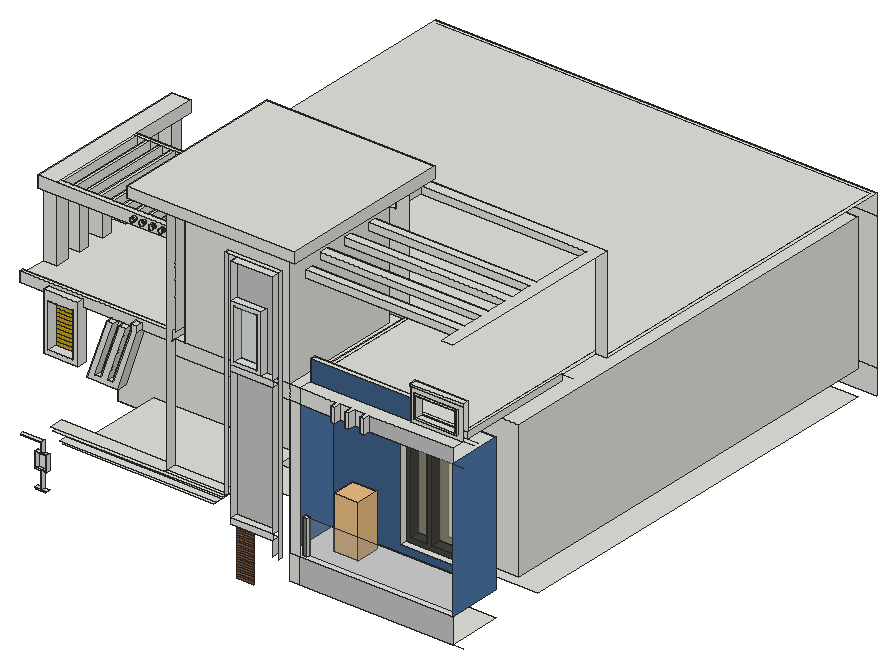
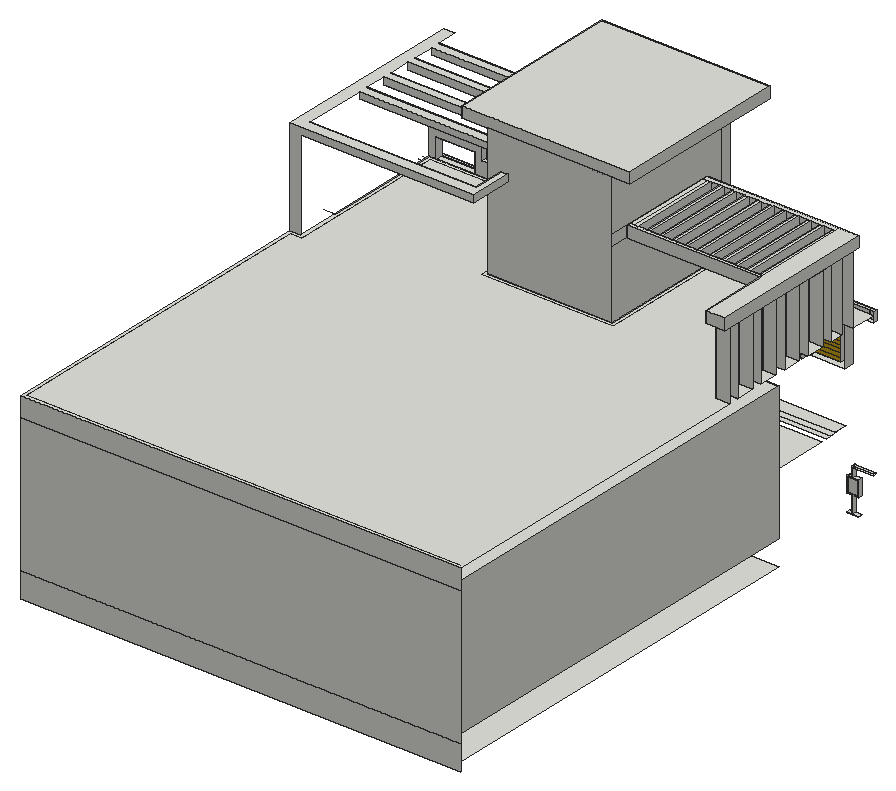
# SketchUp Ruby script. Lengths in inches.
U = 1.inch
M = Sketchup.active_model
def pt(a) = Geom::Point3d.new(a.map { |v| v * U })
def face(e, loops, mat)
  f = e.add_face(loops[0].map { |a| pt(a) })
  loops[1..].each { |l| e.add_face(l.map { |a| pt(a) }).erase! }
  f.material = f.back_material = mat if mat
  f
end
# faces: each face lists its corners as indices into pts; further lists are holes
def faces(e, pts, list, mat = nil) = list.each { |f| face(e, (f[0].is_a?(Array) ? f : [f]).map { |l| l.map { |i| pts[i] } }, mat) }
# xy, xz, yz: faces in a plane at the given z, y or x. An outline is a flat list of corners, or four numbers for a rectangle; further outlines are holes
def ring(l) = l.size == 4 ? [[l[0], l[1]], [l[2], l[1]], [l[2], l[3]], [l[0], l[3]]] : l.each_slice(2).to_a
def flat(e, list, mat, &to3) = list.each { |f| face(e, (f[0].is_a?(Array) ? f : [f]).map { |l| ring(l).map { |u, v| to3.(u, v) } }, mat) }
def xy(e, z, list, mat = nil) = flat(e, list, mat) { |x, y| [x, y, z] }
def xz(e, y, list, mat = nil) = flat(e, list, mat) { |x, z| [x, y, z] }
def yz(e, x, list, mat = nil) = flat(e, list, mat) { |y, z| [x, y, z] }
def lines(e, pts, list) = list.each { |a, b| e.add_line(pt(pts[a]), pt(pts[b])) }
# prism: a flat outline (further loops are holes) pulled along v
def prism(e, loops, v, mat = nil)
  f = face(e, loops, mat); d = Geom::Vector3d.new(v.map { |x| x * U })
  f.pushpull(f.normal.samedirection?(d) ? d.length : -d.length)
end
def box(e, o, s, mat = nil) = prism(e, [[o, [o[0] + s[0], o[1], o[2]], [o[0] + s[0], o[1] + s[1], o[2]], [o[0], o[1] + s[1], o[2]]]], [0, 0, s[2]], mat)
def at(x, y, z, deg = 0) = Geom::Transformation.translation(pt([x, y, z])) * Geom::Transformation.rotation(ORIGIN, Z_AXIS, deg.degrees)
def axes(o, x, y, z) = Geom::Transformation.new([*x, 0, *y, 0, *z, 0, *pt(o).to_a, 1])
def part(name) = M.definitions.add(name)
# library, detail: a bought-in or finely detailed component or shape, given as its bounding box
def library(name, o, s) = part(name).tap { |d| box(d.entities, o, s) }
def detail(e, o, s) = box(e.add_group.entities, o, s)
def put(e, d, t, mat = nil) = e.add_instance(d, t).tap { |i| i.material = mat if mat }
def group(e, t, mat = nil) = e.add_group.tap { |g| g.transformation = t; g.material = mat if mat }.entities
root = M.entities
M.materials.add("Brick_09_1K").color = [77, 120, 168]
M.materials.add("Brick_09_1K1").color = [62, 96, 135]
M.materials.add("Glass_Basic_01").color = [161, 173, 186]
M.materials["Glass_Basic_01"].alpha = 0.25
M.materials.add("Glass_Mirror_01").color = [188, 186, 154]
M.materials["Glass_Mirror_01"].alpha = 0.57
M.materials.add("Glass_Safety_01").color = [204, 235, 244]
M.materials["Glass_Safety_01"].alpha = 0.25
M.materials.add("M02_Ash_Whisper").color = [196, 196, 196]
M.materials.add("Metal_32_1K").color = [117, 124, 125]
M.materials.add("Metal_Perforated_08_1K").color = [201, 163, 22]
M.materials.add("Wood_Planks_01_1K").color = [69, 67, 63]
M.materials.add("Wood_Veneer_15_1K").color = [132, 88, 57]
c1 = library("Group_2",[-1.28,-0.39,0],[21.22,20.51,48.44])
xy(root,258.42,[[49.51,78,58.4,81]])
xy(root,259.42,[[48.51,78,54,81],[55,78,59.4,81]])
xy(root,262,[[270,81,413,129],[45,174,45,525,261,525,261,174,270,174,270,525,414,525,414,174]])
xy(root,274.21,[[48.51,78,54,81],[55,78,59.4,81]])
xy(root,275.21,[[49.51,78,58.4,81]])
xy(root,284,[[270,81,413,81,413,85.9375,282.79,85.9375,282.79,84.29,278.91,84.29,278.91,87.59,282.79,87.59,282.79,85.9375,413,85.9375,413,129,270,129],[270,152.59,414,525],[45,174,261,525]])
xy(root,287.08,[[49.51,78,58.4,81]])
xy(root,288.08,[[48.51,78,54,81],[55,78,59.4,81]])
xy(root,290,[[329,129,389,135.39]])
xy(root,294,[[333,135.39,347.33,143.99],[351.33,135.39,385,143.99],[333,143.99,347.33,152.59],[351.33,143.99,385,152.59]],"Wood_Planks_01_1K")
xy(root,295.99,[[36,78,54,81]])
xy(root,296.99,[[36,78,54,81],[54,78,55,81]])
xy(root,297.09,[[228.07,69,228.07,75.9,242.32,75.9,242.32,72.3125,244.4,72.3125,244.4,75.9,265,75.9,265,69]])
xy(root,302.09,[[228.07,69,265,75.9]])
xy(root,304,[[84,77.68,209.07,165]])
xy(root,308,[[80,69,213.07,77.68]])
xy(root,310,[[78,69,215.07,75]])
xy(root,314,[[278.91,84.29,282.79,87.59]])
xy(root,316,[[72,69,221.07,75]])
xy(root,318,[[70,69,169.4,81],[169.4,69,223.07,72.06],[169.4,72.06,223.07,81]])
xy(root,365.83,[[98.85,72.19,126.42,81]])
xy(root,370,[[333,135.39,347.33,143.99],[351.33,135.39,385,143.99],[333,143.99,347.33,152.59],[351.33,143.99,385,152.59]],"Wood_Planks_01_1K")
xy(root,370.3,[[106.4,72.19,111.18,77.88],[117.18,72.19,121.96,77.88]])
xy(root,371.59,[[60.8,72.19,91.1,81]])
xy(root,374,[[329,129,389,135.39]])
xy(root,375.59,[[64.8,72.19,87.1,81]])
xy(root,404,[[310.85,75,310.85,81,270,81,270,174,45,174,45,525,261,525,261,174,270,174,270,525,414,525,414,152.59,270,152.59,270,129,413,129,413,81,339.77,81,339.77,75,336.2,75,336.2,81,327.09,81,327.09,75,323.52,75,323.52,81,314.42,81,314.42,75]])
xy(root,414.39,[[64.8,72.19,87.1,81]])
xy(root,415.99,[[116.24,72.19,122.24,77.88],[127.02,72.19,133.02,77.88],[36,77.88,60.8,81],[91.1,77.88,116.24,81],[142.82,77.88,169.4,81]])
xy(root,416.58,[[310.85,75,314.42,75,314.42,81,323.52,81,323.52,75,327.09,75,327.09,81,336.2,81,336.2,75,339.77,75,339.77,81,413,81,413,92.26,367.22,92.26,367.22,93,279,93,279,81,310.85,81],[169.4,81,169.4,201,279,201,279,81,270,81,270,190.34,177.78,190.34,177.78,81],[177.78,81,270,190.34]])
xy(root,417.54,[[228.07,69,265,75.9]])
xy(root,420.58,[[371.22,91,409,92.26]])
xy(root,421.58,[[373.13,91,407.09,97.45]])
xy(root,421.92,[[137.81,72.19,142.82,77.88]])
xy(root,421.99,[[60.8,72.19,91.1,77.88],[39.02,80.9,166.38,80.9,169.4,81,169.4,201,279,201,279,97.45,413,97.45,413,238.37,423,238.37,423,534,36,534,36,238.91,48,238.91,48,229.77,36,229.77,36,213.43,48,213.43,48,204.29,36,204.29,36,187.95,48,187.95,48,178.8125,36,178.8125,36,162.48,48,162.48,48,153.33,36,153.33,36,137,48,137,48,127.86,36,127.86,36,115.39,48,115.39,48,103.39,36,103.39,36,81,39.02,81]])
xy(root,422.54,[[254.04,69,265,75.9]])
xy(root,424.99,[[36,77.88,169.4,77.88,169.4,81,166.38,80.9,39.02,80.9,39.02,81,36,81]])
xy(root,425.54,[[231.07,69,251.04,75.9]])
xy(root,434.58,[[279,93,367.22,97.45]])
xy(root,439.65,[[373.13,91,407.09,97.45]])
xy(root,440.58,[[371.22,91,409,92.26]])
xy(root,444.58,[[367.22,92,413,92.26]])
xy(root,446.58,[[367.22,92,413,97.45]])
xy(root,469.83,[[231.07,69,251.04,75.9]])
xy(root,472.83,[[228.07,69,254.04,75.9]])
xy(root,481.99,[[36,97.39,48,103.39],[[48,97.39,48,115.39,36,115.39,36,127.86,48,127.86,48,137,36,137,36,153.33,48,153.33,48,162.48,36,162.48,36,178.8125,48,178.8125,48,187.95,36,187.95,36,204.29,48,204.29,48,213.43,36,213.43,36,229.77,48,229.77,48,238.91,36,238.91,36,244.66,52.24,244.66,52.24,185.19,169.4,185.19,169.4,97.39],[66.3,101.83,74.2,181.81],[88.26,101.83,96.16,181.81],[121.2,101.83,129.11,181.81],[143.17,101.83,151.07,181.81],[55.31,101.83,63.22,181.81],[77.28,101.83,85.18,181.81],[99.24,101.83,107.14,181.81],[110.22,101.83,118.125,181.81],[132.1875,101.83,140.09,181.81],[154.15,101.83,162.05,181.81]],[36,103.39,48,115.39],[36,127.86,48,137],[36,153.33,48,162.48],
  [36,178.8125,48,187.95],[36,204.29,48,213.43],[36,229.77,48,238.91]])
xy(root,491.99,[[36,97.39,52.24,244.66],[52.24,97.39,169.4,101.83],[52.24,101.83,55.31,181.81],[63.22,101.83,66.3,181.81],[74.2,101.83,77.28,181.81],
  [85.18,101.83,88.26,181.81],[96.16,101.83,99.24,181.81],[107.14,101.83,110.22,181.81],[118.125,101.83,121.2,181.81],[129.11,101.83,132.1875,181.81],
  [140.09,101.83,143.17,181.81],[151.07,101.83,154.15,181.81],[162.05,101.83,165.13,181.81],[165.13,101.83,169.4,181.81],[52.24,181.81,169.4,185.19]])
xy(root,500.58,[[279,87.5,413,95.04],[258.78,113.85,413,121.39],[258.78,140.21,413,147.74],[258.78,166.56,413,174.09],[261.19,201,261.19,238.37,413,238.37,413,228.37,267.08,228.37,267.08,201]])
xy(root,504.43,[[228.07,69,265,75.9]])
xy(root,506.58,[[413,69,423,69,423,238.37,261.19,238.37,261.19,201,267.08,201,267.08,228.37,413,228.37,413,174.09,258.78,174.09,258.78,166.56,413,166.56,413,147.74,258.78,147.74,258.78,140.21,413,140.21,413,121.39,258.78,121.39,258.78,113.85,413,113.85,413,95.04,279,95.04,279,87.5,413,87.5]])
xy(root,509.43,[[223.07,69,270,72.06]])
xy(root,536.58,[[153.78,48.06,153.78,201,169.4,201,169.4,72.06,279,72.06,279,201,301.25,201,301.25,48.06],[169.4,72.06,177.78,201],[177.78,72.06,279,81],[270,81,279,201],[177.78,190.34,270,201]])
xy(root,546.58,[[153.78,48.06,301.25,201]])
xz(root,48.06,[[153.78,536.58,301.25,546.58]])
xz(root,69,[[228.07,297.09,265,302.09],[228.07,417.54,265,422.54],[[228.07,422.54,254.04,472.83],[231.07,425.54,251.04,469.83]]])
xz(root,72.19,[[98.85,365.83,126.42,365.83,142.82,415.99,142.82,421.92,137.81,421.92,137.81,415.99,121.96,370.3,117.18,370.3,133.02,415.99,127.02,415.99,111.18,370.3,106.4,370.3,122.24,415.99,116.24,415.99],[[60.8,371.59,91.1,421.99],[64.8,375.59,87.1,414.39]]])
xz(root,75,[[310.85,404,314.42,416.58],[323.52,404,327.09,416.58],[336.2,404,339.77,416.58]])
xz(root,75.9,[[231.07,425.54,251.04,469.83]],"Glass_Safety_01")
xz(root,75.9,[[228.07,302.09,265,417.54],[254.04,422.54,265,422.54,265,504.43,228.07,504.43,228.07,472.83,254.04,472.83]],"M02_Ash_Whisper")
xz(root,75.9,[[228.07,251.47,242.32,253.37],[228.07,253.37,242.32,255.27],[228.07,255.27,242.32,257.17],[228.07,257.17,242.32,259.08],[228.07,259.08,242.32,260.98],
  [228.07,260.98,242.32,262.88],[228.07,262.88,242.32,264.78],[228.07,264.78,242.32,266.68],[228.07,266.68,242.32,268.58],[228.07,268.58,242.32,270.48],
  [228.07,270.48,242.32,272.38],[228.07,272.38,242.32,274.28],[228.07,274.28,242.32,276.18],[228.07,276.18,242.32,278.09],[228.07,278.09,242.32,279.99],
  [228.07,279.99,242.32,281.89],[228.07,281.89,242.32,283.79],[228.07,283.79,242.32,285.6875],[228.07,285.6875,242.32,287.59],[228.07,287.59,242.32,289.49],
  [228.07,289.49,242.32,291.39],[228.07,291.39,242.32,293.29],[228.07,293.29,242.32,295.19],[228.07,295.19,242.32,297.09]],"Wood_Veneer_15_1K")
xz(root,77.88,[[106.4,370.3,111.18,370.3,127.02,415.99,122.24,415.99],[117.18,370.3,121.96,370.3,137.81,415.99,133.02,415.99],[36,415.99,60.8,415.99,60.8,421.99,91.1,421.99,91.1,415.99,137.81,415.99,137.81,421.92,142.82,421.92,142.82,415.99,169.4,415.99,169.4,424.99,36,424.99]])
xz(root,80.9,[[39.02,421.99,60.8,424.99],[60.8,421.99,91.1,424.99],[91.1,421.99,166.38,424.99]])
xz(root,81,[[270,262,279,284],[49.51,275.21,58.4,287.08],[270,284,279,404],[169.4,404,270,416.58],[270,404,279,416.58],
  [279,404,310.85,416.58],[314.42,404,323.52,416.58],[327.09,404,336.2,416.58],[177.78,416.58,270,536.58],[36,421.99,39.02,424.99]])
xz(root,81,[[279,262,413,284],[339.77,404,413,416.58]],"M02_Ash_Whisper")
xz(root,81,[[64.8,375.59,87.1,378.82],[64.8,378.82,87.1,382.05],[64.8,382.05,87.1,385.29],[64.8,385.29,87.1,388.52],[64.8,388.52,87.1,391.75],
  [64.8,391.75,87.1,394.99],[64.8,394.99,87.1,398.22],[64.8,398.22,87.1,401.45],[64.8,401.45,87.1,404.6875],[64.8,404.6875,87.1,407.92],
  [64.8,407.92,87.1,411.15],[64.8,411.15,87.1,414.39]],"Metal_Perforated_08_1K")
xz(root,84.29,[[278.91,284,282.79,314]],"Metal_32_1K")
xz(root,85.9375,[[282.79,284,413,314]],"Glass_Basic_01")
xz(root,87.5,[[279,500.58,413,506.58]])
xz(root,87.59,[[278.91,284,282.79,314]])
xz(root,91,[[[371.22,420.58,409,440.58],[373.13,421.58,407.09,439.65]]])
xz(root,92,[[367.22,444.58,413,446.58]])
xz(root,92.26,[[[367.22,416.58,413,444.58],[371.22,420.58,409,440.58]]])
xz(root,93,[[279,416.58,367.22,434.58]],"Brick_09_1K1")
xz(root,94.25,[[120.73,485.68,121.23,485.75,121.7,485.9375,122.1,486.25,122.41,486.65,122.6,487.11,122.67,487.61,122.6,488.12,122.41,488.58,122.1,488.98,121.7,489.29,121.23,489.48,120.73,489.55,120.23,489.48,119.76,489.29,119.36,488.98,119.06,488.58,118.86,488.12,118.8,487.61,118.86,487.11,119.06,486.65,119.36,486.25,119.76,485.9375,120.23,485.75],[129.11,485.68,129.61,485.75,130.08,485.9375,130.48,486.25,130.79,486.65,130.98,487.11,131.05,487.61,130.98,488.12,130.79,488.58,130.48,488.98,130.08,489.29,129.61,489.48,129.11,489.55,128.61,489.48,128.14,489.29,127.74,488.98,127.43,488.58,127.24,488.12,127.18,487.61,127.24,487.11,127.43,486.65,127.74,486.25,128.14,485.9375,128.61,485.75],[137.49,485.68,137.99,485.75,138.46,485.9375,138.86,486.25,139.17,486.65,139.36,487.11,139.42,487.61,139.36,488.12,139.17,488.58,138.86,488.98,138.46,489.29,137.99,489.48,137.49,489.55,136.99,489.48,136.52,489.29,136.12,488.98,135.8125,488.58,135.62,488.12,135.55,487.61,135.62,487.11,135.8125,486.65,136.12,486.25,136.52,485.9375,136.99,485.75],[145.87,485.68,146.37,485.75,146.84,485.9375,147.24,486.25,147.54,486.65,147.74,487.11,147.8,487.61,147.74,488.12,147.54,488.58,147.24,488.98,146.84,489.29,146.37,489.48,145.87,489.55,145.37,489.48,144.9,489.29,144.5,488.98,144.19,488.58,144,488.12,143.93,487.61,144,487.11,144.19,486.65,144.5,486.25,144.9,485.9375,145.37,485.75],[154.25,485.68,154.75,485.75,155.21,485.9375,155.61,486.25,155.92,486.65,156.12,487.11,156.18,487.61,156.12,488.12,155.92,488.58,155.61,488.98,155.21,489.29,154.75,489.48,154.25,489.55,153.75,489.48,153.28,489.29,152.88,488.98,152.57,488.58,152.375,488.12,152.3125,487.61,152.375,487.11,152.57,486.65,152.88,486.25,153.28,485.9375,153.75,485.75],
  [162.625,485.68,163.125,485.75,163.59,485.9375,163.99,486.25,164.3,486.65,164.49,487.11,164.56,487.61,164.49,488.12,164.3,488.58,163.99,488.98,163.59,489.29,163.125,489.48,162.625,489.55,162.125,489.48,161.66,489.29,161.26,488.98,160.95,488.58,160.75,488.12,160.6875,487.61,160.75,487.11,160.95,486.65,161.26,486.25,161.66,485.9375,162.125,485.75]])
xz(root,95.04,[[279,500.58,413,506.58]])
xz(root,97.39,[[[36,481.99,169.4,491.99],[120.73,485.68,120.23,485.75,119.76,485.9375,119.36,486.25,119.06,486.65,118.86,487.11,118.8,487.61,118.86,488.12,119.06,488.58,119.36,488.98,119.76,489.29,120.23,489.48,120.73,489.55,121.23,489.48,121.7,489.29,122.1,488.98,122.41,488.58,122.6,488.12,122.67,487.61,122.6,487.11,122.41,486.65,122.1,486.25,121.7,485.9375,121.23,485.75],[129.11,485.68,128.61,485.75,128.14,485.9375,127.74,486.25,127.43,486.65,127.24,487.11,127.18,487.61,127.24,488.12,127.43,488.58,127.74,488.98,128.14,489.29,128.61,489.48,129.11,489.55,129.61,489.48,130.08,489.29,130.48,488.98,130.79,488.58,130.98,488.12,131.05,487.61,130.98,487.11,130.79,486.65,130.48,486.25,130.08,485.9375,129.61,485.75],[137.49,485.68,136.99,485.75,136.52,485.9375,136.12,486.25,135.8125,486.65,135.62,487.11,135.55,487.61,135.62,488.12,135.8125,488.58,136.12,488.98,136.52,489.29,136.99,489.48,137.49,489.55,137.99,489.48,138.46,489.29,138.86,488.98,139.17,488.58,139.36,488.12,139.42,487.61,139.36,487.11,139.17,486.65,138.86,486.25,138.46,485.9375,137.99,485.75],[145.87,485.68,145.37,485.75,144.9,485.9375,144.5,486.25,144.19,486.65,144,487.11,143.93,487.61,144,488.12,144.19,488.58,144.5,488.98,144.9,489.29,145.37,489.48,145.87,489.55,146.37,489.48,146.84,489.29,147.24,488.98,147.54,488.58,147.74,488.12,147.8,487.61,147.74,487.11,147.54,486.65,147.24,486.25,146.84,485.9375,146.37,485.75],[154.25,485.68,153.75,485.75,153.28,485.9375,152.88,486.25,152.57,486.65,152.375,487.11,152.3125,487.61,152.375,488.12,152.57,488.58,152.88,488.98,153.28,489.29,153.75,489.48,154.25,489.55,154.75,489.48,155.21,489.29,155.61,488.98,155.92,488.58,156.12,488.12,156.18,487.61,156.12,487.11,155.92,486.65,155.61,486.25,155.21,485.9375,154.75,485.75],[162.625,485.68,162.125,485.75,161.66,485.9375,161.26,486.25,160.95,486.65,160.75,487.11,160.6875,487.61,160.75,488.12,160.95,488.58,161.26,488.98,161.66,489.29,162.125,489.48,162.625,489.55,163.125,489.48,163.59,489.29,163.99,488.98,164.3,488.58,164.49,488.12,164.56,487.61,164.49,487.11,164.3,486.65,163.99,486.25,163.59,485.9375,163.125,485.75]]])
xz(root,97.45,[[279,416.58,279,421.99,373.13,421.99,373.13,421.58,407.09,421.58,407.09,421.99,413,421.99,413,416.58],[373.13,421.58,407.09,421.99],[279,421.99,279,434.58,367.22,434.58,367.22,446.58,413,446.58,413,421.99,407.09,421.99,407.09,439.65,373.13,439.65,373.13,421.99]])
xz(root,101.83,[[55.31,481.99,63.22,491.99],[66.3,481.99,74.2,491.99],[77.28,481.99,85.18,491.99],[88.26,481.99,96.16,491.99],[99.24,481.99,107.14,491.99],
  [110.22,481.99,118.125,491.99],[121.2,481.99,129.11,491.99],[132.1875,481.99,140.09,491.99],[143.17,481.99,151.07,491.99],[154.15,481.99,162.05,491.99]])
xz(root,103.39,[[36,421.99,48,481.99]])
xz(root,113.85,[[258.78,500.58,413,506.58]])
xz(root,115.39,[[36,421.99,48,481.99]])
xz(root,121.39,[[258.78,500.58,413,506.58]])
xz(root,127.86,[[36,421.99,48,481.99]])
xz(root,129,[[[270,284,413,404],[329,290,389,374]]],"Brick_09_1K1")
xz(root,135.39,[[[329,290,389,374],[351.33,294,385,370],[333,294,347.33,370]]],"Wood_Planks_01_1K")
xz(root,137,[[36,421.99,48,481.99]])
xz(root,140.21,[[258.78,500.58,413,506.58]])
xz(root,143.99,[[333,294,347.33,370],[351.33,294,385,370]],"Glass_Mirror_01")
xz(root,147.74,[[258.78,500.58,413,506.58]])
xz(root,152.59,[[[270,284,414,404],[351.33,294,385,370],[333,294,347.33,370]]])
xz(root,153.33,[[36,421.99,48,481.99]])
xz(root,162.48,[[36,421.99,48,481.99]])
xz(root,166.56,[[258.78,500.58,413,506.58]])
xz(root,174,[[45,284,261,404],[261,284,270,404]])
xz(root,174.09,[[258.78,500.58,413,506.58]])
xz(root,178.8125,[[36,421.99,48,481.99]])
xz(root,181.81,[[55.31,481.99,63.22,491.99],[66.3,481.99,74.2,491.99],[77.28,481.99,85.18,491.99],[88.26,481.99,96.16,491.99],[99.24,481.99,107.14,491.99],
  [110.22,481.99,118.125,491.99],[121.2,481.99,129.11,491.99],[132.1875,481.99,140.09,491.99],[143.17,481.99,151.07,491.99],[154.15,481.99,162.05,491.99]])
xz(root,185.19,[[52.24,481.99,169.4,491.99]])
xz(root,187.95,[[36,421.99,48,481.99]])
xz(root,190.34,[[177.78,416.58,270,536.58]])
xz(root,201,[[169.4,416.58,279,421.99],[[169.4,421.99,279,536.58],[261.19,500.58,267.08,506.58]],[153.78,536.58,301.25,546.58]])
xz(root,204.29,[[36,421.99,48,481.99]])
xz(root,213.43,[[36,421.99,48,481.99]])
xz(root,228.37,[[267.08,500.58,413,506.58]])
xz(root,229.77,[[36,421.99,48,481.99]])
xz(root,238.37,[[413,421.99,413,500.58,261.19,500.58,261.19,506.58,423,506.58,423,421.99]])
xz(root,238.91,[[36,421.99,48,481.99]])
xz(root,244.66,[[36,481.99,52.24,491.99]])
xz(root,525,[[45,284,261,404],[270,284,414,404]])
xz(root,534,[[36,262,423,284],[36,284,423,404],[36,404,423,421.99]])
yz(root,36,[[77.88,415.99,81,424.99],[97.39,481.99,244.66,491.99]])
yz(root,39.02,[[80.9,421.99,81,424.99]])
yz(root,45,[[174,284,525,404]])
yz(root,48,[[103.39,421.99,115.39,481.99],[127.86,421.99,137,481.99],[153.33,421.99,162.48,481.99],[178.8125,421.99,187.95,481.99],[204.29,421.99,213.43,481.99],
  [229.77,421.99,238.91,481.99]])
yz(root,48.51,[[78,274.21,81,288.08]])
yz(root,49.51,[[78,275.21,81,287.08]])
yz(root,52.24,[[185.19,481.99,244.66,491.99]])
yz(root,54,[[78,259.42,81,274.21],[78,288.08,81,295.99]])
yz(root,55,[[78,259.42,81,274.21],[78,288.08,81,296.99]])
yz(root,55.31,[[101.83,481.99,181.81,491.99]])
yz(root,58.4,[[78,275.21,81,287.08]])
yz(root,59.4,[[78,274.21,81,288.08]])
yz(root,60.8,[[72.19,371.59,72.19,421.99,77.88,421.99,77.88,415.99,81,415.99,81,371.59]])
yz(root,63.22,[[101.83,481.99,181.81,491.99]])
yz(root,64.8,[[72.19,375.59,81,414.39]])
yz(root,66.3,[[101.83,481.99,181.81,491.99]])
yz(root,74.2,[[101.83,481.99,181.81,491.99]])
yz(root,77.28,[[101.83,481.99,181.81,491.99]])
yz(root,85.18,[[101.83,481.99,181.81,491.99]])
yz(root,87.1,[[72.19,375.59,81,414.39]])
yz(root,88.26,[[101.83,481.99,181.81,491.99]])
yz(root,91.1,[[72.19,371.59,81,371.59,81,415.99,77.88,415.99,77.88,421.99,72.19,421.99]])
yz(root,96.16,[[101.83,481.99,181.81,491.99]])
yz(root,99.24,[[101.83,481.99,181.81,491.99]])
yz(root,107.14,[[101.83,481.99,181.81,491.99]])
yz(root,110.22,[[101.83,481.99,181.81,491.99]])
yz(root,118.125,[[101.83,481.99,181.81,491.99]])
yz(root,121.2,[[101.83,481.99,181.81,491.99]])
yz(root,129.11,[[101.83,481.99,181.81,491.99]])
yz(root,132.1875,[[101.83,481.99,181.81,491.99]])
yz(root,137.81,[[72.19,415.99,77.88,421.92]])
yz(root,140.09,[[101.83,481.99,181.81,491.99]])
yz(root,142.82,[[72.19,415.99,77.88,421.92]])
yz(root,143.17,[[101.83,481.99,181.81,491.99]])
yz(root,151.07,[[101.83,481.99,181.81,491.99]])
yz(root,153.78,[[48.06,536.58,201,546.58]])
yz(root,154.15,[[101.83,481.99,181.81,491.99]])
yz(root,162.05,[[101.83,481.99,181.81,491.99]])
yz(root,169.4,[[72.06,318,72.06,536.58,81,536.58,81,424.99,77.88,424.99,77.88,415.99,81,415.99,81,318],[77.88,415.99,81,416.58],[77.88,416.58,77.88,424.99,81,424.99,81,421.99,201,421.99,201,416.58],[81,421.99,81,536.58,201,536.58,201,491.99,97.39,491.99,97.39,481.99,201,481.99,201,421.99],[97.39,481.99,185.19,491.99],
  [185.19,481.99,201,491.99]])
yz(root,177.78,[[81,416.58,190.34,536.58]])
yz(root,223.07,[[69,318,72.06,509.43]])
yz(root,228.07,[[69,302.09,75.9,417.54],[69,472.83,75.9,504.43]])
yz(root,231.07,[[69,425.54,75.9,469.83]])
yz(root,251.04,[[69,425.54,75.9,469.83]])
yz(root,254.04,[[69,422.54,75.9,472.83]])
yz(root,258.78,[[113.85,500.58,121.39,506.58],[140.21,500.58,147.74,506.58],[166.56,500.58,174.09,506.58]])
yz(root,261,[[174,284,525,404]])
yz(root,261.19,[[201,500.58,238.37,506.58]])
yz(root,265,[[69,284,75.9,297.09],[69,302.09,75.9,417.54],[69,422.54,75.9,504.43]])
yz(root,267.08,[[201,500.58,228.37,506.58]])
yz(root,270,[[69,284,72.06,509.43],[152.59,284,174,404],[174,284,525,404],[81,416.58,190.34,536.58]])
yz(root,270,[[81,284,129,404]],"Brick_09_1K")
yz(root,278.91,[[84.29,284,87.59,314]])
yz(root,279,[[93,416.58,97.45,434.58],[97.45,416.58,201,421.99]])
yz(root,282.79,[[84.29,284,85.9375,314],[85.9375,284,87.59,314]])
yz(root,301.25,[[48.06,536.58,201,546.58]])
yz(root,310.85,[[75,404,81,416.58]])
yz(root,314.42,[[75,404,81,416.58]])
yz(root,323.52,[[75,404,81,416.58]])
yz(root,327.09,[[75,404,81,416.58]])
yz(root,329,[[129,290,135.39,374]])
yz(root,333,[[135.39,294,143.99,370],[143.99,294,152.59,370]],"Wood_Planks_01_1K")
yz(root,336.2,[[75,404,81,416.58]])
yz(root,339.77,[[75,404,81,416.58]])
yz(root,347.33,[[135.39,294,143.99,370],[143.99,294,152.59,370]],"Wood_Planks_01_1K")
yz(root,351.33,[[135.39,294,143.99,370],[143.99,294,152.59,370]],"Wood_Planks_01_1K")
yz(root,367.22,[[92.26,416.58,93,434.58],[92.26,434.58,92.26,444.58,92,444.58,92,446.58,97.45,446.58,97.45,434.58]])
yz(root,371.22,[[91,420.58,92.26,440.58]])
yz(root,373.13,[[91,421.58,97.45,439.65]])
yz(root,385,[[135.39,294,143.99,370],[143.99,294,152.59,370]],"Wood_Planks_01_1K")
yz(root,389,[[129,290,135.39,374]])
yz(root,407.09,[[91,421.58,97.45,439.65]])
yz(root,409,[[91,420.58,92.26,440.58]])
yz(root,413,[[97.45,416.58,201,421.99]])
yz(root,413,[[81,284,129,404]],"Brick_09_1K")
yz(root,414,[[152.59,284,525,404]])
p = [[116.24,81,415.99],[98.85,81,365.83],[98.85,72.19,365.83],[116.24,72.19,415.99],[116.24,77.88,415.99],[126.42,81,365.83],
  [142.82,81,415.99],[142.82,77.88,415.99],[142.82,72.19,415.99],[126.42,72.19,365.83],[122.24,72.19,415.99],[106.4,72.19,370.3],
  [106.4,77.88,370.3],[122.24,77.88,415.99],[111.18,72.19,370.3],[127.02,72.19,415.99],[127.02,77.88,415.99],[111.18,77.88,370.3],
  [133.02,72.19,415.99],[117.18,72.19,370.3],[117.18,77.88,370.3],[133.02,77.88,415.99],[121.96,72.19,370.3],[137.81,72.19,415.99],
  [137.81,77.88,415.99],[121.96,77.88,370.3],[169.4,81,421.99],[166.38,80.9,421.99],[166.38,80.9,424.99],[169.4,81,424.99],
  [119.76,97.39,485.9375],[120.23,97.39,485.75],[120.23,94.25,485.75],[119.76,94.25,485.9375],[120.73,97.39,485.68],[120.73,94.25,485.68],
  [121.23,97.39,485.75],[121.23,94.25,485.75],[121.7,97.39,485.9375],[121.7,94.25,485.9375],[128.14,97.39,485.9375],[128.61,97.39,485.75],
  [128.61,94.25,485.75],[128.14,94.25,485.9375],[129.11,97.39,485.68],[129.11,94.25,485.68],[129.61,97.39,485.75],[129.61,94.25,485.75],
  [130.08,97.39,485.9375],[130.08,94.25,485.9375],[136.52,97.39,485.9375],[136.99,97.39,485.75],[136.99,94.25,485.75],[136.52,94.25,485.9375],
  [137.49,97.39,485.68],[137.49,94.25,485.68],[137.99,97.39,485.75],[137.99,94.25,485.75],[138.46,97.39,485.9375],[138.46,94.25,485.9375],
  [144.9,97.39,485.9375],[145.37,97.39,485.75],[145.37,94.25,485.75],[144.9,94.25,485.9375],[145.87,97.39,485.68],[145.87,94.25,485.68],
  [146.37,97.39,485.75],[146.37,94.25,485.75],[146.84,97.39,485.9375],[146.84,94.25,485.9375],[153.28,97.39,485.9375],[153.75,97.39,485.75],
  [153.75,94.25,485.75],[153.28,94.25,485.9375],[154.25,97.39,485.68],[154.25,94.25,485.68],[154.75,97.39,485.75],[154.75,94.25,485.75],
  [155.21,97.39,485.9375],[155.21,94.25,485.9375],[161.66,97.39,485.9375],[162.125,97.39,485.75],[162.125,94.25,485.75],[161.66,94.25,485.9375],
  [162.625,97.39,485.68],[162.625,94.25,485.68],[163.125,97.39,485.75],[163.125,94.25,485.75],[163.59,97.39,485.9375],[163.59,94.25,485.9375],
  [119.36,97.39,486.25],[119.36,94.25,486.25],[122.1,97.39,486.25],[122.1,94.25,486.25],[127.74,97.39,486.25],[127.74,94.25,486.25],
  [130.48,97.39,486.25],[130.48,94.25,486.25],[136.12,97.39,486.25],[136.12,94.25,486.25],[138.86,97.39,486.25],[138.86,94.25,486.25],
  [144.5,97.39,486.25],[144.5,94.25,486.25],[147.24,97.39,486.25],[147.24,94.25,486.25],[152.88,97.39,486.25],[152.88,94.25,486.25],
  [155.61,97.39,486.25],[155.61,94.25,486.25],[161.26,97.39,486.25],[161.26,94.25,486.25],[163.99,97.39,486.25],[163.99,94.25,486.25],
  [119.06,97.39,486.65],[119.06,94.25,486.65],[122.41,97.39,486.65],[122.41,94.25,486.65],[127.43,97.39,486.65],[127.43,94.25,486.65],
  [130.79,97.39,486.65],[130.79,94.25,486.65],[135.8125,97.39,486.65],[135.8125,94.25,486.65],[139.17,97.39,486.65],[139.17,94.25,486.65],
  [144.19,97.39,486.65],[144.19,94.25,486.65],[147.54,97.39,486.65],[147.54,94.25,486.65],[152.57,97.39,486.65],[152.57,94.25,486.65],
  [155.92,97.39,486.65],[155.92,94.25,486.65],[160.95,97.39,486.65],[160.95,94.25,486.65],[164.3,97.39,486.65],[164.3,94.25,486.65],
  [118.86,97.39,487.11],[118.86,94.25,487.11],[122.6,97.39,487.11],[122.6,94.25,487.11],[127.24,97.39,487.11],[127.24,94.25,487.11],
  [130.98,97.39,487.11],[130.98,94.25,487.11],[135.62,97.39,487.11],[135.62,94.25,487.11],[139.36,97.39,487.11],[139.36,94.25,487.11],
  [144,97.39,487.11],[144,94.25,487.11],[147.74,97.39,487.11],[147.74,94.25,487.11],[152.375,97.39,487.11],[152.375,94.25,487.11],
  [156.12,97.39,487.11],[156.12,94.25,487.11],[160.75,97.39,487.11],[160.75,94.25,487.11],[164.49,97.39,487.11],[164.49,94.25,487.11],
  [118.8,97.39,487.61],[118.8,94.25,487.61],[122.67,97.39,487.61],[122.67,94.25,487.61],[127.18,97.39,487.61],[127.18,94.25,487.61],
  [131.05,97.39,487.61],[131.05,94.25,487.61],[135.55,97.39,487.61],[135.55,94.25,487.61],[139.42,97.39,487.61],[139.42,94.25,487.61],
  [143.93,97.39,487.61],[143.93,94.25,487.61],[147.8,97.39,487.61],[147.8,94.25,487.61],[152.3125,97.39,487.61],[152.3125,94.25,487.61],
  [156.18,97.39,487.61],[156.18,94.25,487.61],[160.6875,97.39,487.61],[160.6875,94.25,487.61],[164.56,97.39,487.61],[164.56,94.25,487.61],
  [118.86,97.39,488.12],[118.86,94.25,488.12],[122.6,97.39,488.12],[122.6,94.25,488.12],[127.24,97.39,488.12],[127.24,94.25,488.12],
  [130.98,97.39,488.12],[130.98,94.25,488.12],[135.62,97.39,488.12],[135.62,94.25,488.12],[139.36,97.39,488.12],[139.36,94.25,488.12],
  [144,97.39,488.12],[144,94.25,488.12],[147.74,97.39,488.12],[147.74,94.25,488.12],[152.375,97.39,488.12],[152.375,94.25,488.12],
  [156.12,97.39,488.12],[156.12,94.25,488.12],[160.75,97.39,488.12],[160.75,94.25,488.12],[164.49,97.39,488.12],[164.49,94.25,488.12],
  [119.06,97.39,488.58],[119.06,94.25,488.58],[122.41,97.39,488.58],[122.41,94.25,488.58],[127.43,97.39,488.58],[127.43,94.25,488.58],
  [130.79,97.39,488.58],[130.79,94.25,488.58],[135.8125,97.39,488.58],[135.8125,94.25,488.58],[139.17,97.39,488.58],[139.17,94.25,488.58],
  [144.19,97.39,488.58],[144.19,94.25,488.58],[147.54,97.39,488.58],[147.54,94.25,488.58],[152.57,97.39,488.58],[152.57,94.25,488.58],
  [155.92,97.39,488.58],[155.92,94.25,488.58],[160.95,97.39,488.58],[160.95,94.25,488.58],[164.3,97.39,488.58],[164.3,94.25,488.58],
  [119.36,97.39,488.98],[119.36,94.25,488.98],[122.1,97.39,488.98],[122.1,94.25,488.98],[127.74,97.39,488.98],[127.74,94.25,488.98],
  [130.48,97.39,488.98],[130.48,94.25,488.98],[136.12,97.39,488.98],[136.12,94.25,488.98],[138.86,97.39,488.98],[138.86,94.25,488.98],
  [144.5,97.39,488.98],[144.5,94.25,488.98],[147.24,97.39,488.98],[147.24,94.25,488.98],[152.88,97.39,488.98],[152.88,94.25,488.98],
  [155.61,97.39,488.98],[155.61,94.25,488.98],[161.26,97.39,488.98],[161.26,94.25,488.98],[163.99,97.39,488.98],[163.99,94.25,488.98],
  [119.76,97.39,489.29],[119.76,94.25,489.29],[121.7,97.39,489.29],[121.7,94.25,489.29],[128.14,97.39,489.29],[128.14,94.25,489.29],
  [130.08,97.39,489.29],[130.08,94.25,489.29],[136.52,97.39,489.29],[136.52,94.25,489.29],[138.46,97.39,489.29],[138.46,94.25,489.29],
  [144.9,97.39,489.29],[144.9,94.25,489.29],[146.84,97.39,489.29],[146.84,94.25,489.29],[153.28,97.39,489.29],[153.28,94.25,489.29],
  [155.21,97.39,489.29],[155.21,94.25,489.29],[161.66,97.39,489.29],[161.66,94.25,489.29],[163.59,97.39,489.29],[163.59,94.25,489.29],
  [120.23,97.39,489.48],[120.23,94.25,489.48],[121.23,97.39,489.48],[121.23,94.25,489.48],[128.61,97.39,489.48],[128.61,94.25,489.48],
  [129.61,97.39,489.48],[129.61,94.25,489.48],[136.99,97.39,489.48],[136.99,94.25,489.48],[137.99,97.39,489.48],[137.99,94.25,489.48],
  [145.37,97.39,489.48],[145.37,94.25,489.48],[146.37,97.39,489.48],[146.37,94.25,489.48],[153.75,97.39,489.48],[153.75,94.25,489.48],
  [154.75,97.39,489.48],[154.75,94.25,489.48],[162.125,97.39,489.48],[162.125,94.25,489.48],[163.125,97.39,489.48],[163.125,94.25,489.48],
  [120.73,97.39,489.55],[120.73,94.25,489.55],[129.11,97.39,489.55],[129.11,94.25,489.55],[137.49,97.39,489.55],[137.49,94.25,489.55],
  [145.87,97.39,489.55],[145.87,94.25,489.55],[154.25,97.39,489.55],[154.25,94.25,489.55],[162.625,97.39,489.55],[162.625,94.25,489.55],
  [270,174,262],[270,129,262],[265,69,422.54],[265.25,69,422.54],[413,81,262],[423,81,262],
  [423,93,416.58],[413,93,416.58],[423,97.45,416.58],[413,97.45,416.58],[413,81,404],[423,81,404],
  [423,201,421.99],[413,201,421.99],[413,92.26,416.58],[419.98,530.98,421.99],[39.02,530.98,421.99],[166.38,81,421.99],
  [166.38,204.02,421.99],[282.02,204.02,421.99],[282.02,100.47,421.99],[373.13,100.47,421.99],[407.09,100.47,421.99],[409.98,100.47,421.99],
  [409.98,201,421.99],[409.98,241.39,421.99],[419.98,241.39,421.99]]
faces(root,p,[[0,1,2,3,4],[5,6,7,8,9],[10,11,12,13],[14,15,16,17],[18,19,20,21],[22,23,24,25],[26,27,28,29],[30,31,32,33],
  [31,34,35,32],[34,36,37,35],[36,38,39,37],[40,41,42,43],[41,44,45,42],[44,46,47,45],[46,48,49,47],[50,51,52,53],
  [51,54,55,52],[54,56,57,55],[56,58,59,57],[60,61,62,63],[61,64,65,62],[64,66,67,65],[66,68,69,67],[70,71,72,73],
  [71,74,75,72],[74,76,77,75],[76,78,79,77],[80,81,82,83],[81,84,85,82],[84,86,87,85],[86,88,89,87],[90,30,33,91],
  [38,92,93,39],[94,40,43,95],[48,96,97,49],[98,50,53,99],[58,100,101,59],[102,60,63,103],[68,104,105,69],[106,70,73,107],
  [78,108,109,79],[110,80,83,111],[88,112,113,89],[114,90,91,115],[92,116,117,93],[118,94,95,119],[96,120,121,97],[122,98,99,123],
  [100,124,125,101],[126,102,103,127],[104,128,129,105],[130,106,107,131],[108,132,133,109],[134,110,111,135],[112,136,137,113],[138,114,115,139],
  [116,140,141,117],[142,118,119,143],[120,144,145,121],[146,122,123,147],[124,148,149,125],[150,126,127,151],[128,152,153,129],[154,130,131,155],
  [132,156,157,133],[158,134,135,159],[136,160,161,137],[162,138,139,163],[140,164,165,141],[166,142,143,167],[144,168,169,145],[170,146,147,171],
  [148,172,173,149],[174,150,151,175],[152,176,177,153],[178,154,155,179],[156,180,181,157],[182,158,159,183],[160,184,185,161],[186,162,163,187],
  [164,188,189,165],[190,166,167,191],[168,192,193,169],[194,170,171,195],[172,196,197,173],[198,174,175,199],[176,200,201,177],[202,178,179,203],
  [180,204,205,181],[206,182,183,207],[184,208,209,185],[210,186,187,211],[188,212,213,189],[214,190,191,215],[192,216,217,193],[218,194,195,219],
  [196,220,221,197],[222,198,199,223],[200,224,225,201],[226,202,203,227],[204,228,229,205],[230,206,207,231],[208,232,233,209],[234,210,211,235],
  [212,236,237,213],[238,214,215,239],[216,240,241,217],[242,218,219,243],[220,244,245,221],[246,222,223,247],[224,248,249,225],[250,226,227,251],
  [228,252,253,229],[254,230,231,255],[232,256,257,233],[258,234,235,259],[236,260,261,237],[262,238,239,263],[240,264,265,241],[266,242,243,267],
  [244,268,269,245],[270,246,247,271],[248,272,273,249],[274,250,251,275],[252,276,277,253],[278,254,255,279],[256,280,281,257],[282,258,259,283],
  [260,284,285,261],[286,262,263,287],[264,288,289,265],[290,266,267,291],[268,292,293,269],[294,270,271,295],[272,296,297,273],[298,274,275,299],
  [276,300,301,277],[302,278,279,303],[280,304,305,281],[306,282,283,307],[284,306,307,285],[308,286,287,309],[288,308,309,289],[310,290,291,311],
  [292,310,311,293],[312,294,295,313],[296,312,313,297],[314,298,299,315],[300,314,315,301],[316,302,303,317],[304,316,317,305]])
lines(root,p,[[318,319],[320,321],[322,323],[324,325],[326,327],[328,329],[330,331],[325,332],[333,334],[27,335],[335,336],[336,337],
  [337,338],[338,339],[339,340],[340,341],[341,342],[342,343],[343,344],[344,333]])
put(root,c1,at(293.37,102.43,280.98))
